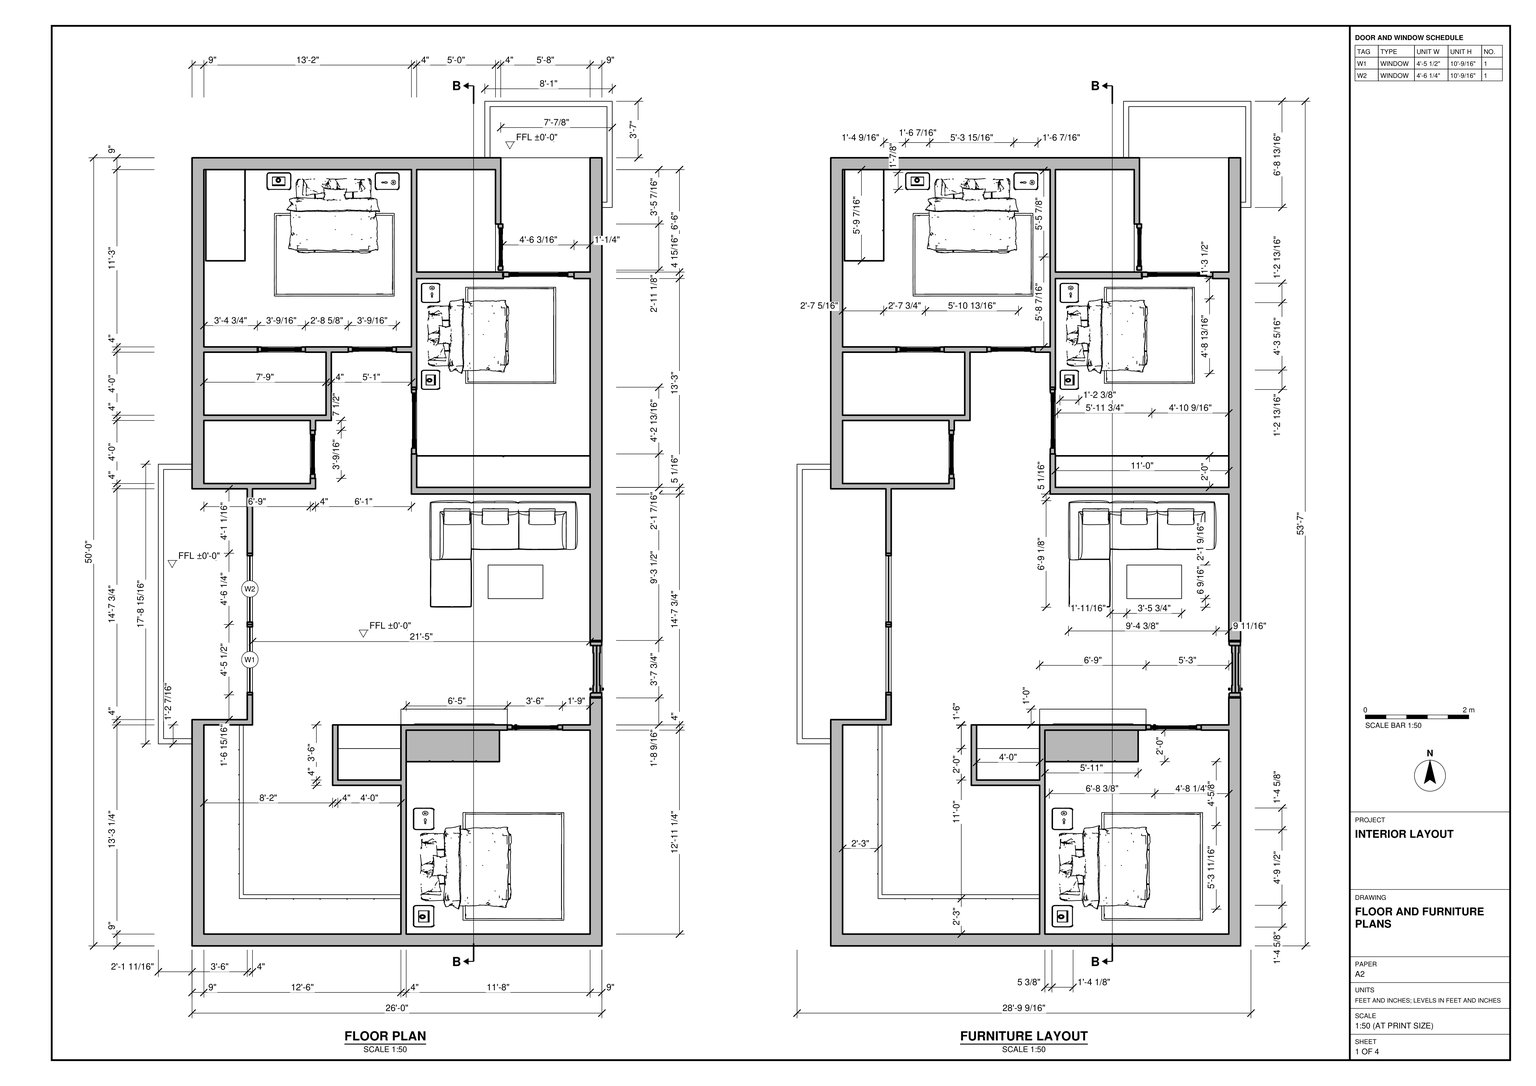
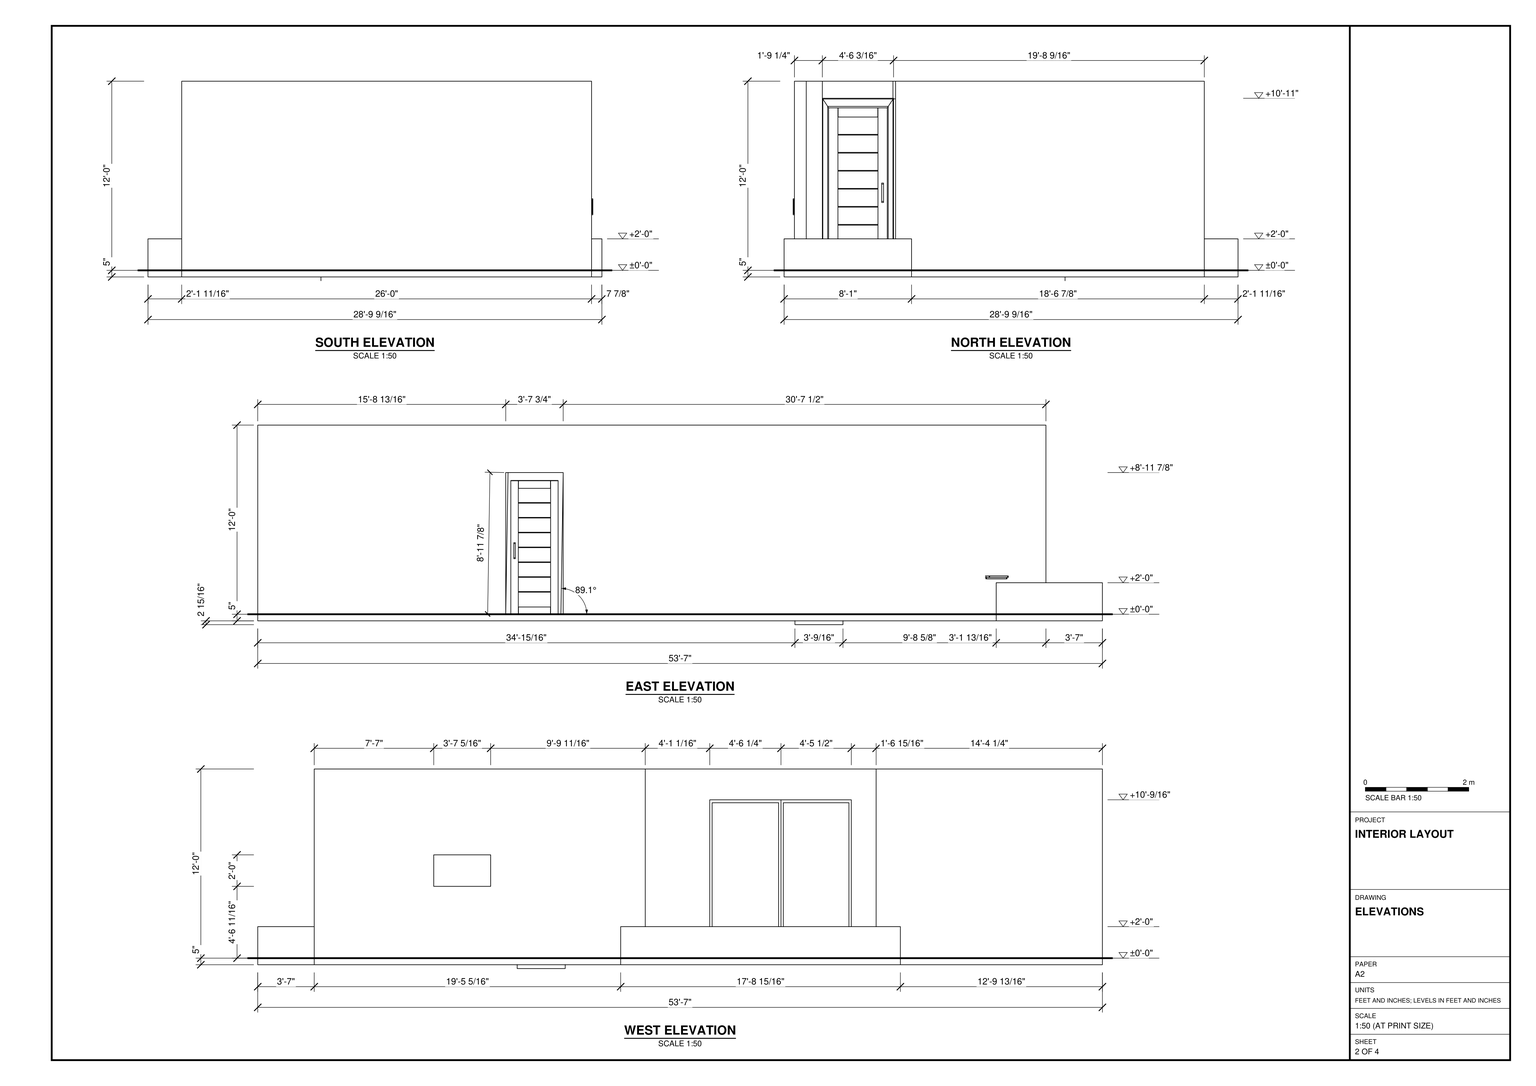
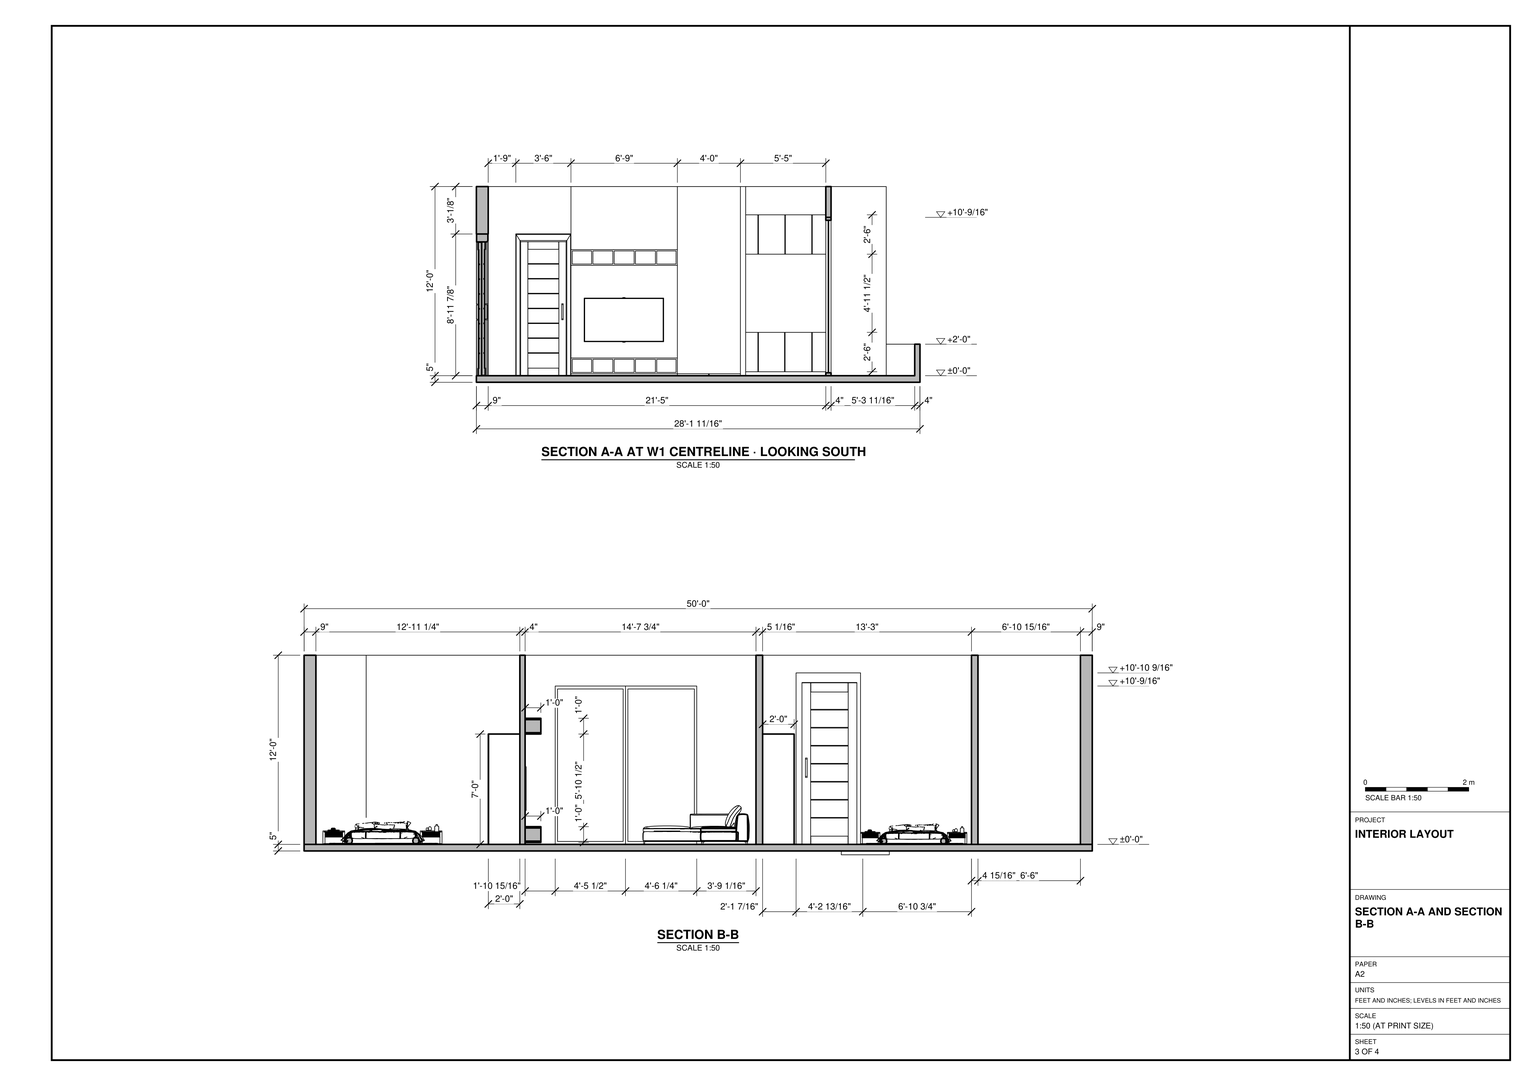
Build the single-storey residential interior shown in task_files/diagram_01.pdf. Work in feet and inches. The complete model extents are 56'-4 1/8" along X, 96'-7 5/16" along Y and 12'-7 15/16" along Z. Set the finished floor at ±0'-0". Use the dimensions on the floor and furniture plans to lay out the rooms and their contents.

Model the floor slab, its projecting areas and their low perimeter walls. Follow the stepped exterior wall line and the partition layout, using 9" and 4" wall thicknesses where marked and the local thicknesses shown elsewhere. Position the doors and window units using the plans, elevations and sections. Place the beds and bedside tables in the northwest, middle east and southeast bedrooms. Fit the storage units against the walls indicated on the furniture plan. In the central living room, place the L-shaped sofa and rectangular coffee table opposite the fitted media unit; use the section to set out its upper and lower shelving.

Keep the shell elements and each furniture or joinery piece in separate groups or components, and use components for repeated parts. Decor and loose items may be any suitable library components. Save one SketchUp model as output_files/furnished_three_bedroom_interior_with_fitted_storage.skp.

# SketchUp Ruby script. Lengths in inches.
U = 1.inch
M = Sketchup.active_model
def pt(a) = Geom::Point3d.new(a.map { |v| v * U })
def face(e, loops, mat)
  f = e.add_face(loops[0].map { |a| pt(a) })
  loops[1..].each { |l| e.add_face(l.map { |a| pt(a) }).erase! }
  f.material = f.back_material = mat if mat
  f
end
# faces: each face lists its corners as indices into pts; further lists are holes
def faces(e, pts, list, mat = nil) = list.each { |f| face(e, (f[0].is_a?(Array) ? f : [f]).map { |l| l.map { |i| pts[i] } }, mat) }
# xy, xz, yz: faces in a plane at the given z, y or x. An outline is a flat list of corners, or four numbers for a rectangle; further outlines are holes
def ring(l) = l.size == 4 ? [[l[0], l[1]], [l[2], l[1]], [l[2], l[3]], [l[0], l[3]]] : l.each_slice(2).to_a
def flat(e, list, mat, &to3) = list.each { |f| face(e, (f[0].is_a?(Array) ? f : [f]).map { |l| ring(l).map { |u, v| to3.(u, v) } }, mat) }
def xy(e, z, list, mat = nil) = flat(e, list, mat) { |x, y| [x, y, z] }
def xz(e, y, list, mat = nil) = flat(e, list, mat) { |x, z| [x, y, z] }
def yz(e, x, list, mat = nil) = flat(e, list, mat) { |y, z| [x, y, z] }
def lines(e, pts, list) = list.each { |a, b| e.add_line(pt(pts[a]), pt(pts[b])) }
# prism: a flat outline (further loops are holes) pulled along v
def prism(e, loops, v, mat = nil)
  f = face(e, loops, mat); d = Geom::Vector3d.new(v.map { |x| x * U })
  f.pushpull(f.normal.samedirection?(d) ? d.length : -d.length)
end
def box(e, o, s, mat = nil) = prism(e, [[o, [o[0] + s[0], o[1], o[2]], [o[0] + s[0], o[1] + s[1], o[2]], [o[0], o[1] + s[1], o[2]]]], [0, 0, s[2]], mat)
def at(x, y, z, deg = 0) = Geom::Transformation.translation(pt([x, y, z])) * Geom::Transformation.rotation(ORIGIN, Z_AXIS, deg.degrees)
def axes(o, x, y, z) = Geom::Transformation.new([*x, 0, *y, 0, *z, 0, *pt(o).to_a, 1])
def part(name) = M.definitions.add(name)
# library, detail: a bought-in or finely detailed component or shape, given as its bounding box
def library(name, o, s) = part(name).tap { |d| box(d.entities, o, s) }
def detail(e, o, s) = box(e.add_group.entities, o, s)
def put(e, d, t, mat = nil) = e.add_instance(d, t).tap { |i| i.material = mat if mat }
def group(e, t, mat = nil) = e.add_group.tap { |g| g.transformation = t; g.material = mat if mat }.entities
root = M.entities
M.materials.add("CROMO PERFIL METALICO").color = [144, 144, 144]
M.materials.add("MADEIRAS PORTAS MOD 4").color = [48, 37, 30]
M.materials.add("Stone Marble").color = [223, 223, 222]
M.materials.add("[0015_Salmon]").color = [61, 61, 61]
M.materials.add("[Color D01]").color = [255, 242, 204]
M.materials.add("[Color F02]").color = [204, 255, 153]
M.materials.add("[Color M02]").color = [198, 198, 198]
M.materials.add("[Color M07]").color = [58, 58, 58]
M.materials.add("[Slate Light Tile]").color = [20, 20, 20]
M.materials.add("[Terrazzo Tile Accent]").color = [252, 249, 244]
M.materials.add("[Translucent Glass Gray]3").color = [128, 128, 128]
M.materials["[Translucent Glass Gray]3"].alpha = 0.3
M.materials.add("[Translucent Glass Sky Reflection]").color = [126, 138, 183]
M.materials["[Translucent Glass Sky Reflection]"].alpha = 0.52
M.materials.add("[Wood Bamboo]").color = [177, 105, 43]
c1 = library("3BHK HOUSE PLAN.dwg",[85.28,57.62,0],[24.58,27.6,0.01])
c2 = library("BED_01",[-66.74,-61.37,0],[192.98,188.94,55.24])
c3 = library("michel-club1",[-34.67,-0.85,-0.13],[126.28,91.17,33.41])
c4 = part("Coffee table \#1")
g1 = group(c4.entities,at(-6.53,0,7.875),"Stone Marble")
xy(g1,0,[[6.69,0.16,31.96,41.57]])
xy(g1,3.9375,[[6.69,0.16,31.96,41.57]])
xz(g1,0,[[6.69,0.16,31.96,3.78]])
xz(g1,41.73,[[6.64,0.12,6.64,3.82,6.69,3.78,6.69,0.16],[6.64,0.12,6.69,0.16,31.96,0.16,32,0.12],[32,0.12,31.96,0.16,31.96,3.78,32,3.82],[6.69,0.16,31.96,3.78],[6.69,3.78,6.64,3.82,32,3.82,31.96,3.78]])
yz(g1,6.53,[[0.12,0.12,0.12,3.82,0.16,3.78,0.16,0.16],[0.12,0.12,0.16,0.16,41.57,0.16,41.62,0.12],[41.62,0.12,41.57,0.16,41.57,3.78,41.62,3.82],[0.16,0.16,41.57,3.78],[0.16,3.78,0.12,3.82,41.62,3.82,41.57,3.78]])
yz(g1,32.12,[[0.16,0.16,41.57,3.78]])
p = [[6.57,0.05,3.89],[6.55,0.08,3.86],[6.55,0.08,0.08],[6.57,0.05,0.05],[6.55,41.65,0.08],[6.57,41.6875,0.05],
  [6.61,0.02,0.08],[6.61,0.02,3.86],[6.61,0.08,0.02],[32.04,0.08,0.02],[32.07,0.05,0.05],[32.04,0.02,0.08],
  [6.61,41.65,0.02],[32.07,0.05,3.89],[32.04,0.02,3.86],[32.04,41.65,0.02],[32.07,41.6875,0.05],[32.1,0.08,0.08],
  [32.1,0.08,3.86],[32.1,41.65,0.08],[6.64,0.12,0.01],[6.69,0.16,0],[31.96,0.16,0],[32,0.12,0.01],
  [6.64,41.62,0.01],[6.69,41.57,0],[31.96,41.57,0],[32,41.62,0.01],[6.55,41.65,3.86],[6.57,41.6875,3.89],
  [6.61,41.71,0.08],[32.04,41.71,0.08],[6.61,41.71,3.86],[32.04,41.71,3.86],[32.07,41.6875,3.89],[32.1,41.65,3.86],
  [6.64,0.01,0.12],[6.64,0.01,3.82],[6.69,0,0.16],[6.69,0,3.78],[32,0.01,0.12],[31.96,0,0.16],
  [32,0.01,3.82],[31.96,0,3.78],[6.53,0.12,3.82],[6.53,0.12,0.12],[6.53,41.62,0.12],[32.11,0.12,0.12],
  [32.12,0.16,0.16],[32.12,0.16,3.78],[32.11,0.12,3.82],[32.11,41.62,0.12],[32.12,41.57,0.16],[6.53,41.62,3.82],
  [32.11,41.62,3.82],[32.12,41.57,3.78],[6.64,41.73,3.82],[6.64,41.73,0.12],[32,41.73,0.12],[32,41.73,3.82],
  [32.04,0.08,3.92],[6.61,0.08,3.92],[6.61,41.65,3.92],[32.04,41.65,3.92],[32,0.12,3.93],[6.64,0.12,3.93],
  [31.96,0.16,3.9375],[6.69,0.16,3.9375],[6.64,41.62,3.93],[6.69,41.57,3.9375],[32,41.62,3.93],[31.96,41.57,3.9375]]
faces(g1,p,[[0,1,2,3],[3,2,4,5],[3,6,7,0],[3,8,9,10],[10,11,6,3],[5,12,8,3],[10,13,14,11],[15,16,10,9],
  [10,17,18,13],[10,16,19,17],[20,21,22,23],[8,20,23,9],[12,24,20,8],[24,25,21,20],[26,27,23,22],[27,15,9,23],
  [12,15,27,24],[24,27,26,25],[28,29,5,4],[5,16,15,12],[5,30,31,16],[5,29,32,30],[16,31,33,34],[19,16,34,35],
  [6,36,37,7],[36,38,39,37],[40,41,38,36],[11,40,36,6],[11,14,42,40],[40,42,43,41],[1,44,45,2],[2,45,46,4],
  [47,48,49,50],[17,47,50,18],[17,19,51,47],[47,51,52,48],[53,28,4,46],[51,19,35,54],[52,51,54,55],[30,32,56,57],
  [30,57,58,31],[31,58,59,33],[43,42,37,39],[37,42,14,7],[1,28,53,44],[50,49,55,54],[18,50,54,35],[59,56,32,33],
  [0,29,28,1],[7,14,13,0],[0,13,60,61],[0,61,62,29],[60,13,34,63],[13,18,35,34],[61,60,64,65],[65,64,66,67],
  [61,65,68,62],[65,67,69,68],[70,64,60,63],[66,64,70,71],[62,68,70,63],[68,69,71,70],[29,62,63,34],[33,32,29,34]])
g2 = group(c4.entities,at(-3.1,3.11,0),"[0015_Salmon]")
xy(g2,-1.18,[[[3.1,-3.11,28.69,38.62],[3.89,-2.32,27.91,37.83]]])
xy(g2,-0.39,[[3.89,-3.11,27.91,-2.32],[3.1,-2.32,3.89,37.83],[27.91,-2.32,28.69,37.83],[3.89,37.83,27.91,38.62]])
xy(g2,7.09,[[3.89,-3.11,3.89,-2.32,3.1,-2.32,3.1,37.83,3.89,37.83,3.89,38.62,27.91,38.62,27.91,37.83,28.69,37.83,28.69,-2.32,27.91,-2.32,27.91,-3.11]])
xy(g2,7.875,[[3.1,-3.11,28.69,38.62]])
xz(g2,-3.11,[[[3.1,-1.18,28.69,7.875],[3.89,-0.39,27.91,7.09]]])
xz(g2,-2.32,[[3.89,-1.18,27.91,-0.39],[3.1,-0.39,3.89,7.09],[27.91,-0.39,28.69,7.09]])
xz(g2,37.83,[[3.89,-1.18,27.91,-0.39],[3.1,-0.39,3.89,7.09],[27.91,-0.39,28.69,7.09]])
xz(g2,38.62,[[[3.1,-1.18,28.69,7.875],[3.89,-0.39,27.91,7.09]]])
yz(g2,3.1,[[[-3.11,-1.18,38.62,7.875],[-2.32,-0.39,37.83,7.09]]])
yz(g2,3.89,[[-2.32,-1.18,37.83,-0.39],[-3.11,-0.39,-2.32,7.09],[37.83,-0.39,38.62,7.09]])
yz(g2,27.91,[[-2.32,-1.18,37.83,-0.39],[-3.11,-0.39,-2.32,7.09],[37.83,-0.39,38.62,7.09]])
yz(g2,28.69,[[[-3.11,-1.18,38.62,7.875],[-2.32,-0.39,37.83,7.09]]])
c5 = part("Coffee table")
put(c5.entities,c4,at(0,0,1.18))
c6 = library("download?mid=50c7180b9fccec56d493bfe20f94b6ab&ctyp=sp&cv=p8.",[149.43,43.83,17.86],[74.75,0.57,42.04])
c7 = part("Group\#13")
xy(c7.entities,0,[[-0.79,16.82,0.71,16.85],[-0.79,16.85,0.71,23.5],[-0.79,23.5,0.71,23.53]],"CROMO PERFIL METALICO")
xy(c7.entities,0.39,[[-0.79,17.125,0.71,23.23]],"CROMO PERFIL METALICO")
xy(c7.entities,1.97,[[-0.79,16.73,0.71,17.125],[-0.79,23.23,0.71,23.62]],"CROMO PERFIL METALICO")
xz(c7.entities,16.73,[[-0.79,0.12,0.71,1.97]],"CROMO PERFIL METALICO")
xz(c7.entities,17.125,[[-0.79,0.39,0.71,1.97]],"CROMO PERFIL METALICO")
xz(c7.entities,23.23,[[-0.79,0.39,0.71,1.97]],"CROMO PERFIL METALICO")
xz(c7.entities,23.62,[[-0.79,0.09,0.71,0.12],[-0.79,0.12,0.71,1.97]],"CROMO PERFIL METALICO")
yz(c7.entities,-0.79,[[16.82,0,16.79,0.02,16.77,0.03,16.75,0.06,16.73,0.12,16.73,1.97,17.125,1.97,17.125,0.39,23.23,0.39,23.23,1.97,23.62,1.97,23.62,0.09,23.61,0.06,23.59,0.03,23.5625,0.02,23.53,0]],"CROMO PERFIL METALICO")
yz(c7.entities,0.71,[[16.82,0,23.53,0,23.5625,0.02,23.59,0.03,23.61,0.06,23.62,0.09,23.62,1.97,23.23,1.97,23.23,0.39,17.125,0.39,17.125,1.97,16.73,1.97,16.73,0.12,16.75,0.06,16.77,0.03,16.79,0.02]],"CROMO PERFIL METALICO")
p = [[-0.79,16.75,0.06],[-0.79,16.77,0.03],[0.71,16.77,0.03],[0.71,16.75,0.06],[-0.79,16.79,0.02],[0.71,16.79,0.02],
  [-0.79,16.82,0],[0.71,16.82,0],[-0.79,23.53,0],[-0.79,23.5625,0.02],[0.71,23.5625,0.02],[0.71,23.53,0],
  [-0.79,23.59,0.03],[0.71,23.59,0.03],[-0.79,23.61,0.06],[0.71,23.61,0.06],[-0.79,16.73,0.12],[-0.79,16.74,0.09],
  [0.71,16.74,0.09],[0.71,16.73,0.12],[-0.79,23.62,0.09],[0.71,23.62,0.09]]
faces(c7.entities,p,[[0,1,2,3],[1,4,5,2],[4,6,7,5],[8,9,10,11],[9,12,13,10],[12,14,15,13],[16,17,18,19],[17,0,3,18],
  [14,20,21,15]],"CROMO PERFIL METALICO")
c8 = part("Framed door panel")
xy(c8.entities,0.21,[[0,0,2.36,0,2.36,7.48,2.17,7.48,2.17,7.64,2.36,7.64,2.36,39.61,2.17,39.61,2.17,39.76,2.36,39.76,2.36,47.24,0,47.24]],"MADEIRAS PORTAS MOD 4")
xy(c8.entities,5.12,[[1.97,7.48,2.17,7.48,2.17,7.64,2.36,7.64,2.36,39.61,2.17,39.61,2.17,39.76,1.97,39.76]],"MADEIRAS PORTAS MOD 4")
xy(c8.entities,15.16,[[1.57,7.48,1.97,39.76]],"MADEIRAS PORTAS MOD 4")
xy(c8.entities,15.55,[[1.57,7.48,1.97,39.76]],"MADEIRAS PORTAS MOD 4")
xy(c8.entities,25.2,[[1.57,7.48,1.97,39.76]],"MADEIRAS PORTAS MOD 4")
xy(c8.entities,25.59,[[1.57,7.48,1.97,39.76]],"MADEIRAS PORTAS MOD 4")
xy(c8.entities,35.24,[[1.57,7.48,1.97,39.76]],"MADEIRAS PORTAS MOD 4")
xy(c8.entities,35.63,[[1.57,7.48,1.97,39.76]],"MADEIRAS PORTAS MOD 4")
xy(c8.entities,45.28,[[1.57,7.48,1.97,39.76]],"MADEIRAS PORTAS MOD 4")
xy(c8.entities,45.67,[[1.57,7.48,1.97,39.76]],"MADEIRAS PORTAS MOD 4")
xy(c8.entities,55.31,[[1.57,7.48,1.97,39.76]],"MADEIRAS PORTAS MOD 4")
xy(c8.entities,55.71,[[1.57,7.48,1.97,39.76]],"MADEIRAS PORTAS MOD 4")
xy(c8.entities,65.35,[[1.57,7.48,1.97,39.76]],"MADEIRAS PORTAS MOD 4")
xy(c8.entities,65.75,[[1.57,7.48,1.97,39.76]],"MADEIRAS PORTAS MOD 4")
xy(c8.entities,75.39,[[1.57,7.48,1.97,39.76]],"MADEIRAS PORTAS MOD 4")
xy(c8.entities,75.79,[[1.57,7.48,1.97,39.76]],"MADEIRAS PORTAS MOD 4")
xy(c8.entities,85.43,[[1.97,7.48,1.97,39.76,2.17,39.76,2.17,39.61,2.36,39.61,2.36,7.64,2.17,7.64,2.17,7.48]],"MADEIRAS PORTAS MOD 4")
xy(c8.entities,90.55,[[0,0,2.36,0,2.36,7.48,2.17,7.48,2.17,7.64,2.36,7.64,2.36,39.61,2.17,39.61,2.17,39.76,2.36,39.76,2.36,47.24,0,47.24]],"MADEIRAS PORTAS MOD 4")
xz(c8.entities,0,[[0,0.21,2.36,90.55]],"MADEIRAS PORTAS MOD 4")
xz(c8.entities,7.48,[[2.17,0.21,2.36,5.12],[1.97,5.12,2.36,15.16],[1.57,15.16,1.57,15.55,1.97,15.55,1.97,25.2,2.36,25.2,2.36,15.16],[1.57,25.2,1.57,25.59,1.97,25.59,1.97,35.24,2.36,35.24,2.36,25.2],[1.57,35.24,1.57,35.63,1.97,35.63,1.97,45.28,2.36,45.28,2.36,35.24],
  [1.57,45.28,1.57,45.67,1.97,45.67,1.97,55.31,2.36,55.31,2.36,45.28],[1.57,55.31,1.57,55.71,1.97,55.71,1.97,65.35,2.36,65.35,2.36,55.31],[1.57,65.35,1.57,65.75,1.97,65.75,1.97,75.39,2.36,75.39,2.36,65.35],[1.57,75.39,1.57,75.79,1.97,75.79,1.97,85.43,2.36,85.43,2.36,75.39],[2.17,85.43,2.36,90.55]],"MADEIRAS PORTAS MOD 4")
xz(c8.entities,7.64,[[2.17,0.21,2.36,5.12],[2.17,85.43,2.36,90.55]],"MADEIRAS PORTAS MOD 4")
xz(c8.entities,39.61,[[2.17,0.21,2.36,5.12],[2.17,85.43,2.36,90.55]],"MADEIRAS PORTAS MOD 4")
xz(c8.entities,39.76,[[2.17,0.21,2.36,5.12],[1.97,5.12,2.36,15.16],[1.57,15.16,2.36,15.16,2.36,25.2,1.97,25.2,1.97,15.55,1.57,15.55],[1.57,25.2,2.36,25.2,2.36,35.24,1.97,35.24,1.97,25.59,1.57,25.59],[1.57,35.24,2.36,35.24,2.36,45.28,1.97,45.28,1.97,35.63,1.57,35.63],
  [1.57,45.28,2.36,45.28,2.36,55.31,1.97,55.31,1.97,45.67,1.57,45.67],[1.57,55.31,2.36,55.31,2.36,65.35,1.97,65.35,1.97,55.71,1.57,55.71],[1.57,65.35,2.36,65.35,2.36,75.39,1.97,75.39,1.97,65.75,1.57,65.75],[1.57,75.39,2.36,75.39,2.36,85.43,1.97,85.43,1.97,75.79,1.57,75.79],[2.17,85.43,2.36,90.55]],"MADEIRAS PORTAS MOD 4")
xz(c8.entities,47.24,[[0,0.21,2.36,90.55]],"MADEIRAS PORTAS MOD 4")
yz(c8.entities,0,[[0,0.21,47.24,90.55]],"MADEIRAS PORTAS MOD 4")
yz(c8.entities,1.57,[[7.48,15.16,39.76,15.55],[7.48,25.2,39.76,25.59],[7.48,35.24,39.76,35.63],[7.48,45.28,39.76,45.67],[7.48,55.31,39.76,55.71],
  [7.48,65.35,39.76,65.75],[7.48,75.39,39.76,75.79]],"MADEIRAS PORTAS MOD 4")
yz(c8.entities,1.97,[[7.48,5.12,39.76,15.16],[7.48,15.55,39.76,25.2],[7.48,25.59,39.76,35.24],[7.48,35.63,39.76,45.28],[7.48,45.67,39.76,55.31],
  [7.48,55.71,39.76,65.35],[7.48,65.75,39.76,75.39],[7.48,75.79,39.76,85.43]],"MADEIRAS PORTAS MOD 4")
yz(c8.entities,2.17,[[7.48,0.21,7.64,5.12],[39.61,0.21,39.76,5.12],[7.48,85.43,7.64,90.55],[39.61,85.43,39.76,90.55]],"MADEIRAS PORTAS MOD 4")
yz(c8.entities,2.36,[[0,0.21,7.48,90.55],[7.64,0.21,39.61,5.12],[39.76,0.21,47.24,90.55],[7.64,85.43,39.61,90.55]],"MADEIRAS PORTAS MOD 4")
put(c8.entities,c7,axes([4.33,43.46,11.46],[0,-1,0],[0,0,1.575],[-1,0,0]))
c9 = part("Framed door panel \#1")
xy(c9.entities,0.21,[[0,0,2.36,0,2.36,7.48,2.17,7.48,2.17,7.64,2.36,7.64,2.36,39.61,2.17,39.61,2.17,39.76,2.36,39.76,2.36,47.24,0,47.24]],"MADEIRAS PORTAS MOD 4")
xy(c9.entities,5.12,[[1.97,7.48,2.17,7.48,2.17,7.64,2.36,7.64,2.36,39.61,2.17,39.61,2.17,39.76,1.97,39.76]],"MADEIRAS PORTAS MOD 4")
xy(c9.entities,15.16,[[1.57,7.48,1.97,39.76]],"MADEIRAS PORTAS MOD 4")
xy(c9.entities,15.55,[[1.57,7.48,1.97,39.76]],"MADEIRAS PORTAS MOD 4")
xy(c9.entities,25.2,[[1.57,7.48,1.97,39.76]],"MADEIRAS PORTAS MOD 4")
xy(c9.entities,25.59,[[1.57,7.48,1.97,39.76]],"MADEIRAS PORTAS MOD 4")
xy(c9.entities,35.24,[[1.57,7.48,1.97,39.76]],"MADEIRAS PORTAS MOD 4")
xy(c9.entities,35.63,[[1.57,7.48,1.97,39.76]],"MADEIRAS PORTAS MOD 4")
xy(c9.entities,45.28,[[1.57,7.48,1.97,39.76]],"MADEIRAS PORTAS MOD 4")
xy(c9.entities,45.67,[[1.57,7.48,1.97,39.76]],"MADEIRAS PORTAS MOD 4")
xy(c9.entities,55.31,[[1.57,7.48,1.97,39.76]],"MADEIRAS PORTAS MOD 4")
xy(c9.entities,55.71,[[1.57,7.48,1.97,39.76]],"MADEIRAS PORTAS MOD 4")
xy(c9.entities,65.35,[[1.57,7.48,1.97,39.76]],"MADEIRAS PORTAS MOD 4")
xy(c9.entities,65.75,[[1.57,7.48,1.97,39.76]],"MADEIRAS PORTAS MOD 4")
xy(c9.entities,75.39,[[1.57,7.48,1.97,39.76]],"MADEIRAS PORTAS MOD 4")
xy(c9.entities,75.79,[[1.57,7.48,1.97,39.76]],"MADEIRAS PORTAS MOD 4")
xy(c9.entities,85.43,[[1.97,7.48,1.97,39.76,2.17,39.76,2.17,39.61,2.36,39.61,2.36,7.64,2.17,7.64,2.17,7.48]],"MADEIRAS PORTAS MOD 4")
xy(c9.entities,90.55,[[0,0,2.36,0,2.36,7.48,2.17,7.48,2.17,7.64,2.36,7.64,2.36,39.61,2.17,39.61,2.17,39.76,2.36,39.76,2.36,47.24,0,47.24]],"MADEIRAS PORTAS MOD 4")
xz(c9.entities,0,[[0,0.21,2.36,90.55]],"MADEIRAS PORTAS MOD 4")
xz(c9.entities,7.48,[[2.17,0.21,2.36,5.12],[1.97,5.12,2.36,15.16],[1.57,15.16,1.57,15.55,1.97,15.55,1.97,25.2,2.36,25.2,2.36,15.16],[1.57,25.2,1.57,25.59,1.97,25.59,1.97,35.24,2.36,35.24,2.36,25.2],[1.57,35.24,1.57,35.63,1.97,35.63,1.97,45.28,2.36,45.28,2.36,35.24],
  [1.57,45.28,1.57,45.67,1.97,45.67,1.97,55.31,2.36,55.31,2.36,45.28],[1.57,55.31,1.57,55.71,1.97,55.71,1.97,65.35,2.36,65.35,2.36,55.31],[1.57,65.35,1.57,65.75,1.97,65.75,1.97,75.39,2.36,75.39,2.36,65.35],[1.57,75.39,1.57,75.79,1.97,75.79,1.97,85.43,2.36,85.43,2.36,75.39],[2.17,85.43,2.36,90.55]],"MADEIRAS PORTAS MOD 4")
xz(c9.entities,7.64,[[2.17,0.21,2.36,5.12],[2.17,85.43,2.36,90.55]],"MADEIRAS PORTAS MOD 4")
xz(c9.entities,39.61,[[2.17,0.21,2.36,5.12],[2.17,85.43,2.36,90.55]],"MADEIRAS PORTAS MOD 4")
xz(c9.entities,39.76,[[2.17,0.21,2.36,5.12],[1.97,5.12,2.36,15.16],[1.57,15.16,2.36,15.16,2.36,25.2,1.97,25.2,1.97,15.55,1.57,15.55],[1.57,25.2,2.36,25.2,2.36,35.24,1.97,35.24,1.97,25.59,1.57,25.59],[1.57,35.24,2.36,35.24,2.36,45.28,1.97,45.28,1.97,35.63,1.57,35.63],
  [1.57,45.28,2.36,45.28,2.36,55.31,1.97,55.31,1.97,45.67,1.57,45.67],[1.57,55.31,2.36,55.31,2.36,65.35,1.97,65.35,1.97,55.71,1.57,55.71],[1.57,65.35,2.36,65.35,2.36,75.39,1.97,75.39,1.97,65.75,1.57,65.75],[1.57,75.39,2.36,75.39,2.36,85.43,1.97,85.43,1.97,75.79,1.57,75.79],[2.17,85.43,2.36,90.55]],"MADEIRAS PORTAS MOD 4")
xz(c9.entities,47.24,[[0,0.21,2.36,90.55]],"MADEIRAS PORTAS MOD 4")
yz(c9.entities,0,[[0,0.21,47.24,90.55]],"MADEIRAS PORTAS MOD 4")
yz(c9.entities,1.57,[[7.48,15.16,39.76,15.55],[7.48,25.2,39.76,25.59],[7.48,35.24,39.76,35.63],[7.48,45.28,39.76,45.67],[7.48,55.31,39.76,55.71],
  [7.48,65.35,39.76,65.75],[7.48,75.39,39.76,75.79]],"MADEIRAS PORTAS MOD 4")
yz(c9.entities,1.97,[[7.48,5.12,39.76,15.16],[7.48,15.55,39.76,25.2],[7.48,25.59,39.76,35.24],[7.48,35.63,39.76,45.28],[7.48,45.67,39.76,55.31],
  [7.48,55.71,39.76,65.35],[7.48,65.75,39.76,75.39],[7.48,75.79,39.76,85.43]],"MADEIRAS PORTAS MOD 4")
yz(c9.entities,2.17,[[7.48,0.21,7.64,5.12],[39.61,0.21,39.76,5.12],[7.48,85.43,7.64,90.55],[39.61,85.43,39.76,90.55]],"MADEIRAS PORTAS MOD 4")
yz(c9.entities,2.36,[[0,0.21,7.48,90.55],[7.64,0.21,39.61,5.12],[39.76,0.21,47.24,90.55],[7.64,85.43,39.61,90.55]],"MADEIRAS PORTAS MOD 4")
put(c9.entities,c7,axes([4.33,3.7,11.46],[0,-1,0],[0,0,1.575],[-1,0,0]))
c10 = part("Agrupar\#1")
xy(c10.entities,0,[[-0.94,0,-1.34,0.39,-1.34,7.48,3.78,7.48,3.78,0.79,2.99,0],[52.125,0,51.34,0.79,51.34,7.48,56.46,7.48,56.46,0.39,56.0625,0]],"MADEIRAS PORTAS MOD 4")
xy(c10.entities,86.77,[[3.78,0.79,51.34,7.09],[3.78,7.09,51.34,7.48]],"MADEIRAS PORTAS MOD 4")
xy(c10.entities,91.89,[[-1.34,0.39,56.46,7.48]],"MADEIRAS PORTAS MOD 4")
xz(c10.entities,0,[[-0.94,0,2.99,0,2.99,87.56,-0.94,91.5],[52.125,0,56.0625,0,56.0625,91.5,52.125,87.56],[2.99,87.56,52.125,87.56,56.0625,91.5,-0.94,91.5]],"MADEIRAS PORTAS MOD 4")
xz(c10.entities,7.48,[[-1.34,0,3.78,0,3.78,86.77,51.34,86.77,51.34,0,56.46,0,56.46,91.89,-1.34,91.89]],"MADEIRAS PORTAS MOD 4")
yz(c10.entities,-1.34,[[0.39,0,7.48,91.89]],"MADEIRAS PORTAS MOD 4")
yz(c10.entities,3.78,[[0.79,0,7.48,86.77]],"MADEIRAS PORTAS MOD 4")
yz(c10.entities,51.34,[[0.79,0,7.09,86.77],[7.09,0,7.48,86.77]],"MADEIRAS PORTAS MOD 4")
yz(c10.entities,56.46,[[0.39,0,7.48,91.89]],"MADEIRAS PORTAS MOD 4")
p = [[-1.34,0.39,0],[-0.94,0,0],[-0.94,0,91.5],[-1.34,0.39,91.89],[3.78,0.79,86.77],[2.99,0,87.56],
  [2.99,0,0],[3.78,0.79,0],[51.34,0.79,0],[52.125,0,0],[52.125,0,87.56],[51.34,0.79,86.77],
  [56.46,0.39,91.89],[56.0625,0,91.5],[56.0625,0,0],[56.46,0.39,0]]
faces(c10.entities,p,[[0,1,2,3],[4,5,6,7],[8,9,10,11],[12,13,14,15],[11,10,5,4],[3,2,13,12]],"MADEIRAS PORTAS MOD 4")
c11 = part("建立群組\#94")
put(c11.entities,c8,axes([2.85,32.65,-0.17],[-0.65909,0,0],[0,-0.62402,0],[0,0,0.82113]),"MADEIRAS PORTAS MOD 4")
put(c11.entities,c9,axes([2.85,3.17,0],[0.65909,0,0],[0,0.62402,0],[0,0,0.82113]),"MADEIRAS PORTAS MOD 4")
put(c11.entities,c10,axes([5.58,0.83,0],[0,0.61989,0],[-0.65909,0,0],[0,0,0.8569]),"MADEIRAS PORTAS MOD 4")
c12 = part("元件\#5")
put(c12.entities,c11,axes([0.98,0,0],[-0.94122,0,0],[0,1,0],[0,0,1.15]))
c13 = part("WINDOW (1)")
xy(c13.entities,0,[[0,0,59.06,1.97]],"[Color M07]")
xy(c13.entities,1.97,[[1.97,0,57.09,0.98],[1.97,0.98,57.09,1.97]],"[Color M07]")
xy(c13.entities,104.33,[[1.97,0,57.09,0.98],[1.97,0.98,57.09,1.97]],"[Color M07]")
xy(c13.entities,106.3,[[0,0,59.06,1.97]],"[Color M07]")
xz(c13.entities,0,[[[0,0,59.06,106.3],[1.97,1.97,57.09,104.33]]],"[Color M07]")
xz(c13.entities,0.98,[[1.97,1.97,57.09,104.33]],"[Translucent Glass Gray]3")
xz(c13.entities,1.97,[[[0,0,59.06,106.3],[1.97,1.97,57.09,104.33]]],"[Color M07]")
yz(c13.entities,0,[[0,0,1.97,106.3]],"[Color M07]")
yz(c13.entities,1.97,[[0,1.97,0.98,104.33],[0.98,1.97,1.97,104.33]],"[Color M07]")
yz(c13.entities,57.09,[[0,1.97,0.98,104.33],[0.98,1.97,1.97,104.33]],"[Color M07]")
yz(c13.entities,59.06,[[0,0,1.97,106.3]],"[Color M07]")
xy(root,5,[[188.6875,140.25,188.6875,164.25,259.6875,164.25,259.6875,140.25,242.1875,140.25,242.1875,140.75,241.6875,140.75,241.6875,140.25,224.4375,140.25,224.4375,140.75,223.9375,140.75,223.9375,140.25,206.6875,140.25,206.6875,140.75,206.1875,140.75,206.1875,140.25]])
xy(root,29,[[136.6875,126.25,184.6875,150.25]])
xy(root,31,[[136.6875,126.25,184.6875,150.25]],"[Terrazzo Tile Accent]")
xy(root,68.5,[[142.16,126.25,178.78,127.25]])
xy(root,71,[[206.1875,140.25,206.6875,140.75],[212.1,140.25,212.6,140.75],[223.9375,140.25,224.4375,140.75],[235.77,140.25,236.27,140.75],[241.6875,140.25,242.1875,140.75]])
xy(root,73.18,[[146.84,126.25,174.1,126.75],[146.84,126.75,174.1,127.25]])
xy(root,74.78,[[148.44,126.25,172.5,126.75]])
xy(root,89,[[188.6875,140.25,206.1875,140.25,206.1875,140.75,206.6875,140.75,206.6875,140.25,223.9375,140.25,223.9375,140.75,224.4375,140.75,224.4375,140.25,241.6875,140.25,241.6875,140.75,242.1875,140.75,242.1875,140.25,259.6875,140.25,259.6875,164.25,188.6875,164.25]],"[Wood Bamboo]")
xy(root,113.4,[[148.44,126.25,172.5,126.75]])
xy(root,115.01,[[146.84,126.25,174.1,126.75],[146.84,126.75,174.1,127.25]])
xy(root,119.6875,[[142.16,126.25,178.78,127.25]])
xz(root,126.25,[[136.6875,29,184.6875,31],[[142.16,68.5,178.78,119.6875],[146.84,73.18,174.1,115.01]],[148.44,74.78,172.5,113.4]])
xz(root,126.75,[[[146.84,73.18,174.1,115.01],[148.44,74.78,172.5,113.4]]])
xz(root,127.25,[[[142.16,68.5,178.78,119.6875],[146.84,73.18,174.1,115.01]]])
xz(root,140.25,[[188.6875,5,206.1875,71],[206.6875,5,223.9375,71],[224.4375,5,241.6875,71],[242.1875,5,259.6875,71],[188.6875,71,206.1875,89],
  [206.6875,71,223.9375,89],[224.4375,71,241.6875,89],[242.1875,71,259.6875,89]],"[Wood Bamboo]")
xz(root,140.75,[[206.1875,5,206.6875,71],[223.9375,5,224.4375,71],[241.6875,5,242.1875,71],[206.1875,71,206.6875,89],[223.9375,71,224.4375,89],
  [241.6875,71,242.1875,89]])
xz(root,150.25,[[136.6875,29,184.6875,31]],"[Terrazzo Tile Accent]")
xz(root,164.25,[[188.6875,5,259.6875,89]])
xz(root,168.25,[[136.6875,6.49,184.6875,149]],"[Translucent Glass Sky Reflection]")
xz(root,180.25,[[185.6875,7.49,200.39,17.49],[201.39,7.49,216.59,17.49],[217.59,7.49,232.79,17.49],[233.79,7.49,248.99,17.49],[249.99,7.49,264.6875,17.49],
  [185.6875,90,200.39,100],[201.39,90,216.59,100],[217.59,90,232.79,100],[233.79,90,248.99,100],[249.99,90,264.6875,100]],"[Translucent Glass Sky Reflection]")
yz(root,136.6875,[[126.25,29,150.25,31]])
yz(root,142.16,[[126.25,68.5,127.25,119.6875]])
yz(root,146.84,[[126.25,73.18,126.75,115.01],[126.75,73.18,127.25,115.01]])
yz(root,148.44,[[126.25,74.78,126.75,113.4]])
yz(root,172.5,[[126.25,74.78,126.75,113.4]])
yz(root,174.1,[[126.25,73.18,126.75,115.01],[126.75,73.18,127.25,115.01]])
yz(root,178.78,[[126.25,68.5,127.25,119.6875]])
yz(root,184.6875,[[126.25,29,150.25,31]])
yz(root,188.6875,[[140.25,5,164.25,89]])
yz(root,206.1875,[[140.25,5,140.75,71],[140.25,71,140.75,89]])
yz(root,206.6875,[[140.25,5,140.75,71],[140.25,71,140.75,89]])
yz(root,223.9375,[[140.25,5,140.75,71],[140.25,71,140.75,89]])
yz(root,224.4375,[[140.25,5,140.75,71],[140.25,71,140.75,89]])
yz(root,241.6875,[[140.25,5,140.75,71],[140.25,71,140.75,89]])
yz(root,242.1875,[[140.25,5,140.75,71],[140.25,71,140.75,89]])
yz(root,259.6875,[[140.25,5,164.25,89]],"[Wood Bamboo]")
p = [[235.77,140.75,5],[235.77,140.75,71],[236.27,140.75,5],[236.27,140.75,71],[212.6,140.75,5],[212.6,140.75,71],
  [212.1,140.75,5],[212.1,140.75,71],[71.6875,330,5],[71.6875,348,5],[113.6875,348,5]]
lines(root,p,[[0,1],[2,3],[4,5],[6,7],[8,9],[9,10]])
put(root,c1,axes([-590.1875,121.43,0],[5.36916,0,0],[0,5.611,0],[0,0,1]))
put(root,c2,axes([134.63,542.49,5],[0.78,0,0],[0,0.78,0],[0,0,0.78]))
put(root,c2,axes([250.48,465.34,5],[0,0.62607,0],[-0.84927,0,0],[0,0,0.52611]))
put(root,c2,axes([250.42,61.11,5],[0,0.7012,0],[-0.95118,0,0],[0,0,0.58924]))
put(root,c3,axes([237.49,258.58,4.99],[0.89,0,0],[0,0.89,0],[0,0,0.89]))
put(root,c5,at(292.79,264.375,5,90))
put(root,c6,axes([376.69,204.21,16],[-0.81,0,0],[0,-0.81,0],[0,0,0.81]))
put(root,c12,axes([336.84,188.78,5],[1.85818,0,0],[0,1.22092,0],[0,0,1.19129]))
put(root,c12,axes([195.95,374.52,4.5625],[0.74445,0,0],[0,1.41785,0],[0,0,1.44668]))
put(root,c12,axes([118.95,355.91,4.5625],[0.74445,0,0],[0,1.02054,0],[0,0,1.44668]))
put(root,c12,axes([144.61,452.73,5],[0,-0.74445,0],[1.02054,0,0],[0,0,1.44668]))
put(root,c12,axes([75.41,452.73,5],[0,-0.74445,0],[1.02054,0,0],[0,0,1.36525]))
put(root,c12,axes([261.95,514.46,4.5625],[0.74445,0,0],[0,0.97979,0],[0,0,1.44668]))
put(root,c12,axes([265.6875,165.21,5],[0,-0.69369,0],[1.17231,0,0],[0,0,1.1927]))
put(root,c12,axes([262.23,509.73,5],[0,-0.74445,0],[1.51307,0,0],[0,0,1.44668]))
put(root,c13,axes([71.6875,244.68,5],[0,0.91833,0],[-2.032,0,0],[0,0,1.13418]))
put(root,c13,axes([71.6875,191.16,5],[0,0.90623,0],[-2.032,0,0],[0,0,1.13418]))
g3 = group(root,at(25.6875,0,0),"[Slate Light Tile]")
xy(g3,0,[[0,0,0,153.79,-25.6875,153.79,-25.6875,366.71,0,366.71,0,600,222.85,600,222.85,643,319.875,643,319.875,562.16,312,562.16,312,0]])
xy(g3,5,[[0,0,312,0,312,566.16,308,566.16,308,4,4,4,4,157.79,0,157.79],[4,4,308,4,308,566.16,315.875,566.16,315.875,639,226.85,639,226.85,596,4,596,4,362.71,-21.6875,362.71,-21.6875,157.79,4,157.79],[0,362.71,4,362.71,4,596,226.85,596,226.85,600,0,600]])
xy(g3,29,[[-25.6875,153.79,0,153.79,0,157.79,-21.6875,157.79,-21.6875,362.71,0,362.71,0,366.71,-25.6875,366.71],[312,562.16,319.875,562.16,319.875,643,222.85,643,222.85,600,226.85,600,226.85,639,315.875,639,315.875,566.16,312,566.16]])
xz(g3,0,[[0,0,312,5]])
xz(g3,153.79,[[-25.6875,0,0,29]])
xz(g3,157.79,[[-21.6875,5,0,29]])
xz(g3,362.71,[[-21.6875,5,0,29]])
xz(g3,366.71,[[-25.6875,0,0,29]])
xz(g3,562.16,[[312,0,319.875,29]])
xz(g3,566.16,[[312,5,315.875,29]])
xz(g3,600,[[0,0,222.85,5],[222.85,5,226.85,29]])
xz(g3,639,[[226.85,5,315.875,29]])
xz(g3,643,[[222.85,0,319.875,29]])
yz(g3,-25.6875,[[153.79,0,366.71,29]])
yz(g3,-21.6875,[[157.79,5,362.71,29]])
yz(g3,0,[[0,0,153.79,5],[366.71,0,600,5],[153.79,5,157.79,29],[362.71,5,366.71,29]])
yz(g3,222.85,[[600,0,643,29]])
yz(g3,226.85,[[600,5,639,29]])
yz(g3,312,[[0,0,562.16,5],[562.16,5,566.16,29]])
yz(g3,315.875,[[566.16,5,639,29]])
yz(g3,319.875,[[562.16,0,643,29]])
g4 = group(root,at(25.6875,0,-2.92),"[Color D01]")
xy(g4,7.92,[[50.28,452,86.28,456]])
xy(g4,62.59,[[0,465.69,9,509.02]])
xy(g4,86.59,[[0,465.69,9,509.02]])
xy(g4,115.8,[[303,190.52,312,232.52]])
xy(g4,115.92,[[240,164.25,282,168.25]])
xy(g4,128.49,[[42,191.16,46,298.91]])
xy(g4,131.55,[[50.28,452,86.28,456]])
xy(g4,138.49,[[90,355.91,94,392.47],[167,374.52,171,423.58],[118.92,452,155.48,456],[231,513,235,549.5625]])
xy(g4,151.92,[[[0,0,312,0,312,600,303,600,303,513,290.75,513,290.75,508.0625,303,508.0625,303,349.0625,171,349.0625,171,508.0625,237,508.0625,237,513,235,513,235,600,0,600,0,348,42,348,42,172.25,0,172.25],[9,9,9,168.25,46,168.25,46,348,94,348,94,400,106,400,106,452,167,452,167,344,303,344,303,168.25,159,168.25,159,126.25,111,126.25,111,168.25,107,168.25,107,122.25,159,122.25,159,9],[163,9,303,164.25],[9,456,167,591],[171,513,231,591],[9,404,102,452],[9,352,90,400]]])
xz(g4,0,[[0,7.92,312,151.92]])
xz(g4,9,[[9,7.92,159,151.92],[163,7.92,303,151.92]])
xz(g4,122.25,[[107,7.92,159,151.92]])
xz(g4,126.25,[[111,7.92,159,151.92]])
xz(g4,164.25,[[163,7.92,165,151.92],[165,7.92,240,7.92,240,115.92,282,115.92,282,7.92,303,7.92,303,151.92,165,151.92]])
xz(g4,168.25,[[9,7.92,12,151.92],[12,7.92,46,151.92],[107,7.92,111,151.92],[159,7.92,159,151.92,303,151.92,303,7.92,282,7.92,282,115.92,240,115.92,240,7.92]])
xz(g4,172.25,[[0,7.92,42,151.92]])
xz(g4,191.16,[[42,7.92,46,128.49]])
xz(g4,298.91,[[42,7.92,46,128.49]])
xz(g4,344,[[167,7.92,303,151.92]])
xz(g4,348,[[0,7.92,42,151.92],[46,7.92,94,151.92]])
xz(g4,349.0625,[[171,7.92,303,151.92]])
xz(g4,352,[[9,7.92,90,151.92]])
xz(g4,355.91,[[90,7.92,94,138.49]])
xz(g4,374.52,[[167,7.92,171,138.49]])
xz(g4,392.47,[[90,7.92,94,138.49]])
xz(g4,400,[[9,7.92,90,151.92],[94,7.92,106,151.92]])
xz(g4,404,[[9,7.92,102,151.92]])
xz(g4,423.58,[[167,7.92,171,138.49]])
xz(g4,452,[[9,7.92,50.28,7.92,50.28,131.55,86.28,131.55,86.28,7.92,102,7.92,102,151.92,9,151.92],[106,7.92,118.92,7.92,118.92,138.49,155.48,138.49,155.48,7.92,167,7.92,167,151.92,106,151.92]])
xz(g4,456,[[9,7.92,9,151.92,167,151.92,167,7.92,155.48,7.92,155.48,138.49,118.92,138.49,118.92,7.92,86.28,7.92,86.28,131.55,50.28,131.55,50.28,7.92]])
xz(g4,465.69,[[0,62.59,9,86.59]])
xz(g4,508.0625,[[171,7.92,237,151.92],[290.75,7.92,303,151.92]])
xz(g4,509.02,[[0,62.59,9,86.59]])
xz(g4,513,[[171,7.92,231,151.92],[231,7.92,231,138.49,235,138.49,235,151.92,237,151.92,237,7.92],[290.75,7.92,303,151.92]])
xz(g4,549.5625,[[231,7.92,235,138.49]])
xz(g4,591,[[9,7.92,167,151.92],[171,7.92,231,151.92]])
xz(g4,600,[[0,7.92,235,151.92],[303,7.92,312,151.92]])
yz(g4,0,[[0,7.92,172.25,151.92],[[348,7.92,600,151.92],[465.69,62.59,509.02,86.59]]])
yz(g4,9,[[9,7.92,168.25,151.92],[352,7.92,400,151.92],[404,7.92,447.62,151.92],[447.62,7.92,452,151.92],[[456,7.92,591,151.92],[465.69,62.59,509.02,86.59]]])
yz(g4,42,[[172.25,7.92,172.25,151.92,348,151.92,348,7.92,298.91,7.92,298.91,128.49,191.16,128.49,191.16,7.92]])
yz(g4,46,[[168.25,7.92,191.16,7.92,191.16,128.49,298.91,128.49,298.91,7.92,348,7.92,348,151.92,168.25,151.92]])
yz(g4,50.28,[[452,7.92,456,131.55]])
yz(g4,86.28,[[452,7.92,456,131.55]])
yz(g4,90,[[352,7.92,352,151.92,400,151.92,400,7.92,392.47,7.92,392.47,138.49,355.91,138.49,355.91,7.92]])
yz(g4,94,[[348,7.92,355.91,7.92,355.91,138.49,392.47,138.49,392.47,7.92,400,7.92,400,151.92,348,151.92]])
yz(g4,102,[[404,7.92,452,151.92]])
yz(g4,106,[[408.94,0,445.5,7.92],[400,7.92,452,151.92]])
yz(g4,107,[[122.25,7.92,168.25,151.92]])
yz(g4,111,[[126.25,7.92,168.25,151.92]])
yz(g4,118.92,[[452,7.92,456,138.49]])
yz(g4,155.48,[[452,7.92,456,138.49]])
yz(g4,159,[[9,7.92,122.25,151.92],[126.25,7.92,168.25,151.92]])
yz(g4,163,[[9,7.92,47.25,151.92],[47.25,7.92,164.25,151.92]])
yz(g4,167,[[344,7.92,348,151.92],[348,7.92,348,151.92,452,151.92,452,7.92,423.58,7.92,423.58,138.49,374.52,138.49,374.52,7.92],[456,7.92,591,151.92]])
yz(g4,171,[[349.0625,7.92,374.52,7.92,374.52,138.49,423.58,138.49,423.58,7.92,508.0625,7.92,508.0625,151.92,349.0625,151.92],[513,7.92,591,151.92]])
yz(g4,231,[[549.5625,7.92,549.5625,138.49,513,138.49,513,151.92,591,151.92,591,7.92]])
yz(g4,235,[[549.5625,7.92,600,7.92,600,151.92,513,151.92,513,138.49,549.5625,138.49]])
yz(g4,237,[[508.0625,7.92,513,151.92]])
yz(g4,240,[[164.25,7.92,168.25,115.92]])
yz(g4,282,[[164.25,7.92,168.25,115.92]])
yz(g4,290.75,[[508.0625,7.92,513,151.92]])
yz(g4,303,[[9,7.92,164.25,151.92],[168.25,7.92,168.25,151.92,344,151.92,344,7.92,230.78,7.92,232.52,115.8,190.52,115.8,188.78,7.92],[349.0625,7.92,508.0625,151.92],[513,7.92,600,151.92]])
yz(g4,312,[[0,7.92,188.78,7.92,190.52,115.8,232.52,115.8,230.78,7.92,600,7.92,600,151.92,0,151.92]])
p = [[303,188.78,7.92],[303,190.52,115.8],[312,190.52,115.8],[312,188.78,7.92],[303,232.52,115.8],[303,230.78,7.92],
  [312,230.78,7.92],[312,232.52,115.8],[282,164.25,7.92],[240,164.25,7.92],[42,191.16,7.92],[42,298.91,7.92],
  [90,355.91,7.92],[90,392.47,7.92],[171,374.52,7.92],[171,423.58,7.92],[231,549.5625,7.92],[231,513,7.92],
  [118.92,456,7.92],[155.48,456,7.92],[303,600,7.92],[235,600,7.92],[237,513,7.92],[290.75,513,7.92]]
faces(g4,p,[[0,1,2,3],[4,5,6,7]])
lines(g4,p,[[3,6],[8,9],[10,11],[12,13],[14,15],[16,17],[18,19],[20,21],[22,23]])
g5 = group(root,at(36.1875,521.5625,5),"[Wood Bamboo]")
xy(g5,0,[[0,0,0,69.4375,29.8125,69.4375,29.8125,46.49,29.3125,46.49,29.3125,46.09,29.8125,46.09,29.8125,23.35,29.3125,23.35,29.3125,22.95,29.8125,22.95,29.8125,0]])
xy(g5,60,[[29.3125,17.16,29.8125,17.56],[29.3125,22.95,29.8125,23.35],[29.3125,34.52,29.8125,34.92],[29.3125,46.09,29.8125,46.49],[29.3125,51.88,29.8125,52.28]])
xy(g5,84,[[0,0,29.8125,0,29.8125,17.16,29.3125,17.16,29.3125,17.56,29.8125,17.56,29.8125,34.52,29.3125,34.52,29.3125,34.92,29.8125,34.92,29.8125,51.88,29.3125,51.88,29.3125,52.28,29.8125,52.28,29.8125,69.4375,0,69.4375]])
xz(g5,0,[[0,0,29.8125,84]])
xz(g5,17.16,[[29.3125,60,29.8125,84]])
xz(g5,17.56,[[29.3125,60,29.8125,84]])
xz(g5,22.95,[[29.3125,0,29.8125,60]])
xz(g5,23.35,[[29.3125,0,29.8125,60]])
xz(g5,34.52,[[29.3125,60,29.8125,84]])
xz(g5,34.92,[[29.3125,60,29.8125,84]])
xz(g5,46.09,[[29.3125,0,29.8125,60]])
xz(g5,46.49,[[29.3125,0,29.8125,60]])
xz(g5,51.88,[[29.3125,60,29.8125,84]])
xz(g5,52.28,[[29.3125,60,29.8125,84]])
xz(g5,69.4375,[[0,0,29.8125,84]])
yz(g5,0,[[0,0,69.4375,84]])
yz(g5,29.3125,[[22.95,0,23.35,60],[46.09,0,46.49,60],[17.16,60,17.56,84],[34.52,60,34.92,84],[51.88,60,52.28,84]])
yz(g5,29.8125,[[0,0,22.95,60],[23.35,0,46.09,60],[46.49,0,69.4375,60],[0,60,17.16,84],[17.56,60,34.52,84],
  [34.92,60,51.88,84],[52.28,60,69.4375,84]])
g6 = group(root,at(34.6875,9,5))
prism(g6,[[[30,159,0],[30,30,0],[150,30,0],[150,0,0],[0,0,0],[0,159,0]]],[0,0,3])
g7 = group(root,at(34.6875,9,8),"[Color M02]")
prism(g7,[[[27,159,0],[27,140.54,0],[26.5,140.54,0],[26.5,140.14,0],[27,140.14,0],[27,121.49,0],[26.5,121.49,0],[26.5,121.09,0],[27,121.09,0],[27,102.63,0],[26.5,102.63,0],[26.5,102.23,0],[27,102.23,0],[27,83.77,0],[26.5,83.77,0],[26.5,83.37,0],[27,83.37,0],[27,64.91,0],[26.5,64.91,0],[26.5,64.51,0],[27,64.51,0],[27,46.06,0],[26.5,46.06,0],[26.5,45.66,0],[27,45.66,0],[27,27,0],[47.3,27,0],[47.3,26.5,0],[47.7,26.5,0],[47.7,27,0],[68,27,0],[68,26.5,0],[68.4,26.5,0],[68.4,27,0],[88.3,27,0],[88.3,26.5,0],[88.7,26.5,0],[88.7,27,0],[108.8,27,0],[108.8,26.5,0],[109.2,26.5,0],[109.2,27,0],[129.3,27,0],[129.3,26.5,0],[129.7,26.5,0],[129.7,27,0],[150,27,0],[150,0,0],[0,0,0],[0,159,0]]],[0,0,30])
g8 = group(root,at(34.6875,9,97.5),"[Color M02]")
prism(g8,[[[27,159,0],[27,140.56,0],[26.5,140.56,0],[26.5,140.16,0],[27,140.16,0],[27,121.66,0],[26.5,121.66,0],[26.5,121.26,0],[27,121.26,0],[27,102.77,0],[26.5,102.77,0],[26.5,102.37,0],[27,102.37,0],[27,83.88,0],[26.5,83.88,0],[26.5,83.48,0],[27,83.48,0],[27,64.99,0],[26.5,64.99,0],[26.5,64.59,0],[27,64.59,0],[27,46.09,0],[26.5,46.09,0],[26.5,45.69,0],[27,45.69,0],[27,27,0],[47.3,27,0],[47.3,26.5,0],[47.7,26.5,0],[47.7,27,0],[67.8,27,0],[67.8,26.5,0],[68.2,26.5,0],[68.2,27,0],[88.3,27,0],[88.3,26.5,0],[88.7,26.5,0],[88.7,27,0],[108.8,27,0],[108.8,26.5,0],[109.2,26.5,0],[109.2,27,0],[129.3,27,0],[129.3,26.5,0],[129.7,26.5,0],[129.7,27,0],[150,27,0],[150,0,0],[0,0,0],[0,159,0]]],[0,0,30])
p = [[27,159.25,0],[27,159.25,30]]
lines(g8,p,[[0,1]])
g9 = group(root,at(136.6875,126.25,5),"[Color F02]")
prism(g9,[[[48,24,0],[48,0,0],[0,0,0],[0,24,0],[23.8,24,0],[23.8,23.5,0],[24.2,23.5,0],[24.2,24,0]]],[0,0,24])
g10 = group(root,at(196.6875,349.0625,5),"[Wood Bamboo]")
xy(g10,0,[[0,0,0,24,65.75,24,65.75,23.5,66.25,23.5,66.25,24,132,24,132,0]])
xy(g10,66,[[65.75,23.5,66.25,24]])
xy(g10,84,[[0,0,132,24]])
xz(g10,0,[[0,0,132,84]])
xz(g10,23.5,[[65.75,0,66.25,66]])
xz(g10,24,[[0,0,65.75,66],[66.25,0,132,66],[0,66,32.75,84],[32.75,66,33.25,84],[33.25,66,65.75,84],
  [65.75,66,66.25,84],[66.25,66,98.75,84],[98.75,66,99.25,84],[99.25,66,132,84]])
yz(g10,0,[[0,0,24,84]])
yz(g10,65.75,[[23.5,0,24,66]])
yz(g10,66.25,[[23.5,0,24,66]])
yz(g10,132,[[0,0,24,84]])
g11 = group(root,at(184.6875,168.25,89),"[Wood Bamboo]")
xy(g11,0,[[0,0,81,12]])
xy(g11,1,[[1,0,15.7,12],[16.7,0,31.9,12],[32.9,0,48.1,12],[49.1,0,64.3,12],[65.3,0,80,12]])
xy(g11,11,[[1,0,15.7,12],[16.7,0,31.9,12],[32.9,0,48.1,12],[49.1,0,64.3,12],[65.3,0,80,12]])
xy(g11,12,[[0,0,81,12]])
xz(g11,0,[[1,1,15.7,11],[16.7,1,31.9,11],[32.9,1,48.1,11],[49.1,1,64.3,11],[65.3,1,80,11]])
xz(g11,12,[[[0,0,81,12],[32.9,1,48.1,11],[49.1,1,64.3,11],[16.7,1,31.9,11],[65.3,1,80,11],[1,1,15.7,11]]])
yz(g11,0,[[0,0,12,12]])
yz(g11,1,[[0,1,12,11]])
yz(g11,15.7,[[0,1,12,11]])
yz(g11,16.7,[[0,1,12,11]])
yz(g11,31.9,[[0,1,12,11]])
yz(g11,32.9,[[0,1,12,11]])
yz(g11,48.1,[[0,1,12,11]])
yz(g11,49.1,[[0,1,12,11]])
yz(g11,64.3,[[0,1,12,11]])
yz(g11,65.3,[[0,1,12,11]])
yz(g11,80,[[0,1,12,11]])
yz(g11,81,[[0,0,12,12]])
p = [[81,0,60],[0,0,60],[81,0,24],[0,0,12],[81,0,12]]
lines(g11,p,[[0,1],[2,0],[1,3],[4,2]])
g12 = group(root,at(184.6875,168.25,6.49),"[Wood Bamboo]")
xy(g12,0,[[0,0,81,12]])
xy(g12,1,[[1,0,15.7,12],[16.7,0,31.9,12],[32.9,0,48.1,12],[49.1,0,64.3,12],[65.3,0,80,12]])
xy(g12,11,[[1,0,15.7,12],[16.7,0,31.9,12],[32.9,0,48.1,12],[49.1,0,64.3,12],[65.3,0,80,12]])
xy(g12,12,[[0,0,81,12]])
xz(g12,0,[[1,1,15.7,11],[16.7,1,31.9,11],[32.9,1,48.1,11],[49.1,1,64.3,11],[65.3,1,80,11]])
xz(g12,12,[[[0,0,81,12],[32.9,1,48.1,11],[49.1,1,64.3,11],[16.7,1,31.9,11],[65.3,1,80,11],[1,1,15.7,11]]])
yz(g12,0,[[0,0,12,12]])
yz(g12,1,[[0,1,12,11]])
yz(g12,15.7,[[0,1,12,11]])
yz(g12,16.7,[[0,1,12,11]])
yz(g12,31.9,[[0,1,12,11]])
yz(g12,32.9,[[0,1,12,11]])
yz(g12,48.1,[[0,1,12,11]])
yz(g12,49.1,[[0,1,12,11]])
yz(g12,64.3,[[0,1,12,11]])
yz(g12,65.3,[[0,1,12,11]])
yz(g12,80,[[0,1,12,11]])
yz(g12,81,[[0,0,12,12]])
p = [[81,0,24],[81,0,60],[0,0,60],[0,0,12],[81,0,12]]
lines(g12,p,[[0,1],[2,3],[4,0]])
